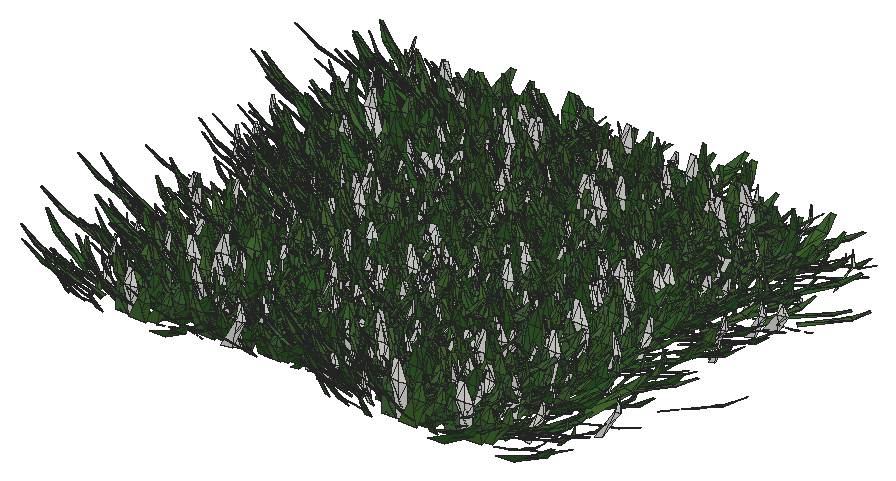
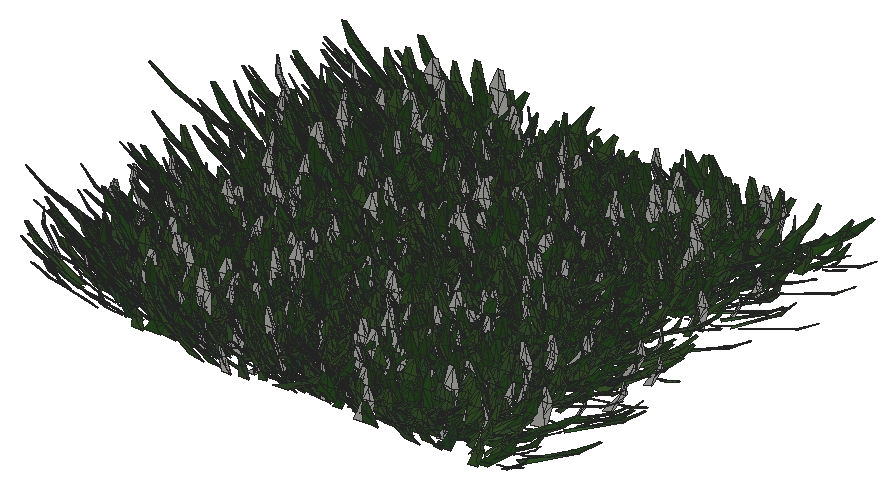
# SketchUp Ruby script. Lengths in inches.
U = 1.inch
M = Sketchup.active_model
def pt(a) = Geom::Point3d.new(a.map { |v| v * U })
def face(e, loops, mat)
  f = e.add_face(loops[0].map { |a| pt(a) })
  loops[1..].each { |l| e.add_face(l.map { |a| pt(a) }).erase! }
  f.material = f.back_material = mat if mat
  f
end
# faces: each face lists its corners as indices into pts; further lists are holes
def faces(e, pts, list, mat = nil) = list.each { |f| face(e, (f[0].is_a?(Array) ? f : [f]).map { |l| l.map { |i| pts[i] } }, mat) }
# xy, xz, yz: faces in a plane at the given z, y or x. An outline is a flat list of corners, or four numbers for a rectangle; further outlines are holes
def ring(l) = l.size == 4 ? [[l[0], l[1]], [l[2], l[1]], [l[2], l[3]], [l[0], l[3]]] : l.each_slice(2).to_a
def flat(e, list, mat, &to3) = list.each { |f| face(e, (f[0].is_a?(Array) ? f : [f]).map { |l| ring(l).map { |u, v| to3.(u, v) } }, mat) }
def xy(e, z, list, mat = nil) = flat(e, list, mat) { |x, y| [x, y, z] }
def xz(e, y, list, mat = nil) = flat(e, list, mat) { |x, z| [x, y, z] }
def yz(e, x, list, mat = nil) = flat(e, list, mat) { |y, z| [x, y, z] }
def lines(e, pts, list) = list.each { |a, b| e.add_line(pt(pts[a]), pt(pts[b])) }
# prism: a flat outline (further loops are holes) pulled along v
def prism(e, loops, v, mat = nil)
  f = face(e, loops, mat); d = Geom::Vector3d.new(v.map { |x| x * U })
  f.pushpull(f.normal.samedirection?(d) ? d.length : -d.length)
end
def box(e, o, s, mat = nil) = prism(e, [[o, [o[0] + s[0], o[1], o[2]], [o[0] + s[0], o[1] + s[1], o[2]], [o[0], o[1] + s[1], o[2]]]], [0, 0, s[2]], mat)
def at(x, y, z, deg = 0) = Geom::Transformation.translation(pt([x, y, z])) * Geom::Transformation.rotation(ORIGIN, Z_AXIS, deg.degrees)
def axes(o, x, y, z) = Geom::Transformation.new([*x, 0, *y, 0, *z, 0, *pt(o).to_a, 1])
def part(name) = M.definitions.add(name)
# library, detail: a bought-in or finely detailed component or shape, given as its bounding box
def library(name, o, s) = part(name).tap { |d| box(d.entities, o, s) }
def detail(e, o, s) = box(e.add_group.entities, o, s)
def put(e, d, t, mat = nil) = e.add_instance(d, t).tap { |i| i.material = mat if mat }
def group(e, t, mat = nil) = e.add_group.tap { |g| g.transformation = t; g.material = mat if mat }.entities
root = M.entities
M.materials.add("Material10").color = [48, 100, 38]
M.materials.add("Material3").color = [68, 110, 58]
M.materials.add("Material4").color = [48, 90, 38]
M.materials.add("Material5").color = [68, 110, 48]
M.materials.add("Material6").color = [48, 90, 48]
M.materials.add("Material7").color = [58, 110, 58]
M.materials.add("Material8").color = [58, 90, 38]
M.materials.add("Material9").color = [68, 100, 58]
c1 = part("grass00")
p = [[-0.6875,0.15,0],[-0.56,0.08,5.52],[-0.04,0.03,2.76],[0.48,-0.02,0],[0.35,-0.02,5.52],[-0.1,-0.14,5.52],
  [-0.12,0.65,8.37],[-0.42,0.65,8.37]]
faces(c1.entities,p,[[0,1,2,3],[3,2,4],[1,5,2],[5,4,2],[1,6,5],[4,5,6],[7,6,1]])
c2 = part("Group16\#1")
put(c2.entities,c1,axes([1.44,-0.61,-0.01],[0.05352,0.12609,0],[-0.10704,0.04543,0.07239],[0.06664,-0.02828,0.11628]),"Material6")
put(c2.entities,c1,axes([0.76,-0.15,-0.01],[0.04676,0.24062,0],[-0.23162,0.04501,0.06642],[0.0652,-0.01267,0.23595]),"Material3")
put(c2.entities,c1,axes([0.79,0.01,-0.01],[-0.00606,0.34651,0],[-0.34381,-0.00602,0.0432],[0.04319,0.00076,0.34386]))
put(c2.entities,c1,axes([1,0.23,-0.01],[-0.07192,0.31144,0],[-0.28722,-0.06632,0.1236],[0.12043,0.02781,0.29478]),"Material5")
put(c2.entities,c1,axes([1.66,0.77,-0.01],[-0.13828,0.29651,0],[-0.21551,-0.1005,0.22471],[0.20365,0.09498,0.23779]),"Material10")
put(c2.entities,c1,axes([0.6875,0.52,-0.01],[-0.18126,0.24051,0],[-0.22746,-0.17142,0.09788],[0.07817,0.05891,0.28481]),"Material5")
put(c2.entities,c1,axes([0.68,0.78,-0.01],[-0.215,0.18688,0],[-0.12385,-0.14248,0.21334],[0.13995,0.16101,0.18878]),"Material3")
put(c2.entities,c1,axes([0.56,1,-0.01],[-0.13756,0.07624,0],[-0.06159,-0.11112,0.0927],[0.04494,0.08108,0.12705]),"Material5")
put(c2.entities,c1,axes([0.2,0.64,-0.01],[-0.23729,0.07254,0],[-0.05711,-0.18681,0.153],[0.04473,0.14632,0.19535]),"Material10")
put(c2.entities,c1,axes([0.0625,0.72,-0.01],[-0.28874,0.02525,0],[-0.02179,-0.24916,0.14647],[0.01276,0.14591,0.25012]),"Material3")
put(c2.entities,c1,axes([-0.08,0.62,-0.01],[-0.34089,-0.04187,0],[0.03255,-0.26504,0.216],[-0.02633,0.21439,0.26703]),"Material10")
put(c2.entities,c1,axes([-0.34,0.98,-0.01],[-0.14314,-0.0493,0],[0.04397,-0.12769,0.06843],[-0.02228,0.0647,0.13505]),"Material10")
put(c2.entities,c1,axes([-0.87,1.45,-0.01],[-0.23488,-0.14114,0],[0.13761,-0.22901,0.06087],[-0.03135,0.05217,0.26717]))
put(c2.entities,c1,axes([-0.72,0.77,-0.01],[-0.14208,-0.13251,0],[0.07209,-0.0773,0.16301],[-0.11118,0.11922,0.1057]),"Material10")
put(c2.entities,c1,axes([-0.62,0.43,-0.01],[-0.14845,-0.21203,0],[0.18654,-0.13061,0.12304],[-0.10079,0.07057,0.22772]),"Material3")
put(c2.entities,c1,axes([-0.68,0.29,-0.01],[-0.13639,-0.32136,0],[0.31723,-0.13464,0.05579],[-0.05136,0.0218,0.34462]),"Material4")
put(c2.entities,c1,axes([-0.64,0.125,-0.01],[-0.0458,-0.23569,0],[0.22124,-0.043,0.08276],[-0.08124,0.01579,0.22538]),"Material7")
put(c2.entities,c1,axes([-1.6,-0.03,-0.01],[0.00576,-0.32897,0],[0.27526,0.00482,0.18018],[-0.18015,-0.00315,0.2753]),"Material5")
put(c2.entities,c1,axes([-1.36,-0.31,-0.01],[0.05718,-0.24765,0],[0.18172,0.04196,0.17267],[-0.16825,-0.03885,0.1865]),"Material10")
put(c2.entities,c1,axes([-1.54,-0.72,-0.01],[0.06537,-0.14017,0],[0.13555,0.06321,0.03939],[-0.0357,-0.01665,0.14956]))
put(c2.entities,c1,axes([-1.19,-0.9,-0.01],[0.09597,-0.12735,0],[0.11214,0.08451,0.07557],[-0.06035,-0.04548,0.14042]),"Material9")
put(c2.entities,c1,axes([-0.47,-0.54,-0.01],[0.11588,-0.10072,0],[0.0618,0.0711,0.12124],[-0.07953,-0.0915,0.0942]))
put(c2.entities,c1,axes([-0.47,-0.84,-0.01],[0.11927,-0.0661,0],[0.06603,0.11913,0.00646],[-0.00313,-0.00565,0.13621]),"Material5")
put(c2.entities,c1,axes([-0.38,-1.24,-0.01],[0.28037,-0.08571,0],[0.0618,0.20215,0.20315],[-0.05939,-0.19428,0.21139]),"Material9")
put(c2.entities,c1,axes([-0.06,-0.66,-0.01],[0.22719,-0.01987,0],[0.01247,0.14255,0.17758],[-0.01547,-0.17691,0.1431]),"Material8")
put(c2.entities,c1,axes([0.11,-0.89,-0.01],[0.14882,0.01828,0],[-0.01058,0.08611,0.12229],[0.01491,-0.12138,0.08676]),"Material6")
put(c2.entities,c1,axes([0.25,-0.72,-0.01],[0.20481,0.07053,0],[-0.06206,0.18022,0.10291],[0.03351,-0.0973,0.1906]),"Material6")
put(c2.entities,c1,axes([0.85,-1.42,-0.01],[0.16481,0.09904,0],[-0.09472,0.15762,0.05616],[0.02893,-0.04814,0.18389]),"Material5")
put(c2.entities,c1,axes([1.01,-1.09,-0.01],[0.21858,0.20385,0],[-0.17495,0.1876,0.15339],[0.10462,-0.11218,0.25652]),"Material10")
put(c2.entities,c1,axes([1.01,-0.71,-0.01],[0.08733,0.12473,0],[-0.06445,0.04512,0.13037],[0.1068,-0.07477,0.07867]),"Material6")
c3 = part("Group15\#1")
put(c3.entities,c2,at(0,0,0))
c4 = part("3darcstudiotree_grass00\#1")
put(c4.entities,c3,at(0,0,0))
put(root,c4,axes([888.68,894.13,0],[0.61281,-1.25792,0],[4.16429,0.12679,-0.0324],[0.1815,0.00553,1.47946]))
put(root,c4,axes([889.35,933.24,0],[-4.67365,-0.16733,0],[0.64986,-1.13441,-0.00988],[0.00864,-0.01508,1.76639]))
put(root,c4,axes([887.89,919.82,0],[-0.28726,1.27917,0],[-3.62125,-0.05083,-0.00552],[-0.03584,-0.0005,1.47331]))
put(root,c4,axes([889.7,899.66,0],[1.5261,-1.19927,0],[4.79938,0.38171,-0.00448],[0.02429,0.00193,1.79011]))
put(root,c4,axes([889.46,902.48,0],[-0.47435,-1.1855,0],[4.17095,-0.10431,-0.05423],[0.34983,-0.00875,1.69842]))
put(root,c4,axes([889.79,918.5,0],[-3.66287,-0.10914,0],[0.53272,-1.11739,-0.01308],[0.00905,-0.01898,1.64432]))
put(root,c4,axes([889.9,927.1,0],[-4.43451,0.03772,0],[-0.16554,-1.21627,-0.01213],[-0.00253,-0.01859,1.86653]))
put(root,c4,axes([889.75,911.6,0],[-3.65887,0.1299,0],[-0.61787,-1.08767,-0.00819],[-0.00564,-0.00993,1.3463]))
put(root,c4,axes([889.55,905.01,0],[-3.669,0.60681,0],[-2.27303,-0.85898,-0.03289],[-0.10969,-0.04145,1.55622]))
put(root,c4,axes([890.45,931.35,0],[-4.28497,-0.45872,0],[1.95501,-1.14138,-0.00601],[0.01191,-0.00695,1.5624]))
put(root,c4,axes([890.35,908.66,0],[-3.05739,-0.71664,0],[2.47729,-0.66055,-0.04465],[0.23187,-0.06183,1.71883]))
put(root,c4,axes([890.83,895.05,0],[-4.36075,-0.60413,0],[2.40015,-1.0828,-0.02403],[0.07228,-0.03261,1.92026]))
put(root,c4,axes([888.54,915.54,0],[3.04221,0.50388,0],[-2.77722,1.04797,-0.00365],[-0.00864,0.00326,1.34685]))
put(root,c4,axes([889.4375,925.43,0],[4.61314,0.2073,0],[-0.8279,1.1515,-0.00017],[-0.00019,0.00026,1.78268]))
put(root,c4,axes([891.2,898.44,0],[-2.44705,-0.6793,0],[3.03744,-0.68387,-0.04825],[0.26014,-0.05857,1.85346]))
put(root,c4,axes([890.42,923.9,0],[-2.92283,0.91805,0],[-3.29129,-0.65491,-0.02078],[-0.1142,-0.02272,1.84714]))
put(root,c4,axes([889.58,905.98,0],[4.43029,0.19931,0],[-0.91399,1.26978,-0.01866],[-0.01759,0.02444,1.717]))
put(root,c4,axes([889.93,921.08,0],[3.52512,0.8325,0],[-3.53899,0.93659,-0.01632],[-0.05093,0.01348,1.46423]))
put(root,c4,axes([890.42,916.13,0],[3.74573,0.67429,0],[-2.32637,0.8077,-0.02682],[-0.11092,0.03851,1.76121]))
put(root,c4,axes([891.78,930.35,0],[-1.7815,0.94038,0],[-4.05374,-0.47998,-0.05633],[-0.34181,-0.04047,1.88219]))
put(root,c4,axes([891.42,913.95,0],[2.43331,0.85712,0],[-3.60269,0.63924,-0.0048],[-0.0225,0.00399,1.58899]))
put(root,c4,axes([893.59,904.56,0],[-3.5004,-0.31733,0],[1.33107,-0.91766,-0.00444],[0.00863,-0.00595,1.39182]))
put(root,c4,axes([894.39,922.36,0],[0.98634,-0.98273,0],[4.96113,0.31121,-0.03647],[0.15012,0.00942,1.35653]))
put(root,c4,axes([894.27,931.77,0],[1.5516,-0.99587,0],[4.11909,0.4011,-0.0174],[0.07644,0.00744,1.30214]))
put(root,c4,axes([894.18,913.87,0],[1.28741,-1.026,0],[3.77436,0.296,-0.02865],[0.19326,0.01516,1.74795]))
put(root,c4,axes([893.8,903.46,0],[2.57556,-0.96136,0],[3.42516,0.57352,-0.05113],[0.25858,0.0433,1.56833]))
put(root,c4,axes([894.82,900.16,0],[0.62856,-1.17531,0],[4.83812,0.16171,-0.0102],[0.05862,0.00196,1.76846]))
put(root,c4,axes([895.13,907.88,0],[-3.61051,-0.41144,0],[1.52061,-0.83398,-0.0331],[0.09259,-0.05078,1.54531]))
put(root,c4,axes([893.88,905.65,0],[2.93142,0.86988,0],[-2.89804,0.61038,-0.04423],[-0.19713,0.04152,1.38013]))
put(root,c4,axes([895.13,921.54,0],[2.02846,-0.79273,0],[3.7574,0.60091,-0.02581],[0.12575,0.02011,1.61243]))
put(root,c4,axes([895.68,915.18,0],[-0.79202,-1.12645,0],[4.16541,-0.18305,-0.04893],[0.31505,-0.01384,1.72817]))
put(root,c4,axes([895.39,930.26,0],[-4.0818,0.563,0],[-2.02545,-0.91779,-0.01481],[-0.0392,-0.01776,1.43556]))
put(root,c4,axes([894.68,924.47,0],[4.56829,-0.12289,0],[0.55043,1.27888,-0.03237],[0.01647,0.03827,1.52951]))
put(root,c4,axes([896.36,901.64,0],[-4.66423,-0.46806,0],[1.3813,-0.8603,-0.04034],[0.1029,-0.06409,1.58691]))
put(root,c4,axes([896.29,919.56,0],[-0.8253,-1.0659,0],[3.55539,-0.17205,-0.00678],[0.0454,-0.0022,1.54322]))
put(root,c4,axes([896.8,917.01,0],[-2.41791,-1.09567,0],[4.13972,-0.57097,-0.0117],[0.05943,-0.0082,1.7149]))
put(root,c4,axes([895.04,932.84,0],[1.31705,0.88702,0],[-3.52607,0.32722,-0.04291],[-0.24696,0.02292,1.44315]))
put(root,c4,axes([895.89,927.84,0],[2.84794,-0.83805,0],[3.51838,0.74728,-0.02612],[0.12969,0.02754,1.8801]))
put(root,c4,axes([895.27,895.97,0],[-0.36246,1.18288,0],[-4.29439,-0.08224,-0.03234],[-0.22764,-0.00436,1.90052]))
put(root,c4,axes([894.93,917.92,0],[4.24178,0.73433,0],[-2.3441,0.84628,-0.05103],[-0.19051,0.06878,1.6877]))
put(root,c4,axes([895.36,896.54,0],[4.6373,-0.30696,0],[1.13066,1.06758,-0.03329],[0.04185,0.03952,1.35616]))
put(root,c4,axes([896.33,898.9375,0],[-3.30831,0.84443,0],[-3.70005,-0.906,-0.0181],[-0.07733,-0.01894,1.93624]))
put(root,c4,axes([897.11,909.39,0],[1.24763,-0.92182,0],[4.38061,0.37056,-0.02846],[0.12558,0.01062,1.34635]))
put(root,c4,axes([897.625,910.63,0],[1.57584,-0.93457,0],[3.47629,0.36635,-0.03331],[0.19752,0.02082,1.51731]))
put(root,c4,axes([897.64,925.62,0],[-2.4775,0.7659,0],[-2.94091,-0.59457,-0.00747],[-0.03328,-0.00673,1.35493]))
put(root,c4,axes([897.78,929.1875,0],[0.67051,0.95222,0],[-4.84197,0.21309,-0.06022],[-0.34411,0.01514,1.78296]))
put(root,c4,axes([897.8,911.56,0],[2.1541,0.73783,0],[-3.48209,0.63537,-0.05552],[-0.23217,0.04236,1.39481]))
put(root,c4,axes([899.92,932.08,0],[-1.49369,-1.06151,0],[3.72951,-0.32799,-0.03242],[0.16562,-0.01457,1.33794]))
put(root,c4,axes([901.23,895.25,0],[-4.2486,-0.47023,0],[1.56425,-0.88333,-0.0129],[0.02854,-0.01611,1.31952]))
put(root,c4,axes([900.17,922.18,0],[-3.0514,0.75193,0],[-3.33727,-0.84644,-0.00446],[-0.01526,-0.00387,1.44777]))
put(root,c4,axes([901.21,913.16,0],[-4.92331,0.15002,0],[-0.48598,-0.99677,-0.03065],[-0.02921,-0.05991,1.97713]))
put(root,c4,axes([901.76,929.9375,0],[-1.91157,-1.00019,0],[4.33506,-0.51782,-0.00689],[0.03608,-0.00431,1.74288]))
put(root,c4,axes([901.7,926.82,0],[-3.45228,-0.31834,0],[1.71903,-1.16515,-0.02933],[0.05627,-0.03814,1.72129]))
put(root,c4,axes([900.31,932.9,0],[4.75785,0.13927,0],[-0.57992,1.23828,-0.02723],[-0.01633,0.03486,1.60719]))
put(root,c4,axes([900.73,898.41,0],[4.24363,-0.133,0],[0.6088,1.21409,-0.03701],[0.03003,0.05988,1.99511]))
put(root,c4,axes([900.46,917.24,0],[4.38323,0.5518,0],[-2.13593,1.06042,-0.03278],[-0.09357,0.04645,1.8841]))
put(root,c4,axes([901.91,912.36,0],[1.80526,-0.93773,0],[4.63497,0.55769,-0.06017],[0.29336,0.0353,1.73941]))
put(root,c4,axes([901.75,905.75,0],[2.55214,-0.79924,0],[2.90871,0.58051,-0.01018],[0.05177,0.01033,1.51436]))
put(root,c4,axes([900.92,924.17,0],[3.99552,0.1688,0],[-0.66851,0.98901,-0.04218],[-0.052,0.07693,1.85529]))
put(root,c4,axes([902.54,902.82,0],[-1.20745,-0.91696,0],[4.5972,-0.37835,-0.05688],[0.32578,-0.02681,1.82396]))
put(root,c4,axes([900.85,909.42,0],[4.60083,0.27128,0],[-0.99888,1.0588,-0.02883],[-0.04481,0.04749,1.84132]))
put(root,c4,axes([901.9375,901.72,0],[3.15828,-0.63994,0],[3.01444,0.92981,-0.02341],[0.07838,0.02418,1.59067]))
put(root,c4,axes([903.11,918.12,0],[-3.6011,-0.51295,0],[1.91228,-0.83905,-0.01205],[0.03293,-0.01445,1.33255]))
put(root,c4,axes([903.23,904.54,0],[-3.34758,-0.57583,0],[2.35115,-0.85428,-0.02104],[0.0798,-0.02899,1.73448]))
put(root,c4,axes([903.24,925.52,0],[-2.89247,-0.63047,0],[2.79907,-0.8026,-0.03875],[0.16322,-0.0468,1.70607]))
put(root,c4,axes([902.44,907.57,0],[2.73531,-0.60508,0],[3.15346,0.89096,-0.04815],[0.2108,0.05956,1.9649]))
put(root,c4,axes([902.18,928.46,0],[3.9102,0.44615,0],[-1.54008,0.84362,-0.03533],[-0.11802,0.06465,1.86502]))
put(root,c4,axes([903.1,915.37,0],[4.11404,0.2026,0],[-0.94809,1.20329,-0.03192],[-0.02927,0.03715,1.45488]))
put(root,c4,axes([903.49,920.89,0],[-0.49166,1.00113,0],[-4.41418,-0.13549,-0.03564],[-0.21762,-0.00668,1.71014]))
put(root,c4,axes([903.1,899.47,0],[4.50169,0.36178,0],[-1.23301,0.95889,-0.00634],[-0.01342,0.01044,1.74238]))
put(root,c4,axes([904.07,910.4,0],[3.54844,-0.68412,0],[2.53941,0.82322,-0.00737],[0.02478,0.00803,1.42978]))
put(root,c4,axes([903.35,896.59,0],[0.51658,1.03873,0],[-3.86244,0.12005,-0.00588],[-0.03275,0.00102,1.36568]))
put(root,c4,axes([903.26,920,0],[2.79958,0.75017,0],[-3.79275,0.88464,-0.03325],[-0.11995,0.02798,1.59934]))
put(root,c4,axes([905.78,931.97,0],[-3.89596,-0.25813,0],[1.01122,-0.9539,-0.01321],[0.02668,-0.02516,1.9444]))
put(root,c4,axes([906.1,909.61,0],[-1.738,-0.84913,0],[4.25665,-0.54453,-0.02541],[0.1,-0.01279,1.32108]))
put(root,c4,axes([905.89,921.55,0],[0.41155,-0.92389,0],[4.43873,0.12358,-0.00391],[0.01942,0.00054,1.39627]))
put(root,c4,axes([905.66,917.17,0],[0.3191,-1.2505,0],[4.37865,0.06983,-0.05413],[0.27394,0.00437,1.39055]))
put(root,c4,axes([905.87,907.09,0],[0.66073,-1.27721,0],[5.08368,0.16437,-0.05291],[0.21846,0.00706,1.33374]))
put(root,c4,axes([906.14,901.94,0],[-4.56571,-0.14579,0],[0.54682,-1.07027,-0.0157],[0.01423,-0.02784,1.92971]))
put(root,c4,axes([906.22,930.68,0],[0.35405,-1.11937,0],[4.05484,0.08016,-0.00365],[0.02209,0.00044,1.54435]))
put(root,c4,axes([906.28,915.22,0],[2.95951,-0.93197,0],[4.0202,0.79789,-0.06314],[0.20058,0.03981,1.30132]))
put(root,c4,axes([906.46,900.2,0],[-3.85049,0.40649,0],[-1.93296,-1.14436,-0.01449],[-0.02989,-0.0177,1.64714]))
put(root,c4,axes([907.85,933.38,0],[-2.15911,-0.91358,0],[4.38085,-0.64709,-0.05519],[0.27113,-0.04005,1.81465]))
put(root,c4,axes([905.8125,910.7,0],[2.25416,0.91391,0],[-3.32067,0.5119,-0.00763],[-0.0422,0.0065,1.58363]))
put(root,c4,axes([906.26,919.56,0],[4.35171,-0.00299,0],[0.0127,1.15651,-0.02008],[0.00031,0.02806,1.61638]))
put(root,c4,axes([906.39,903.58,0],[0.76881,0.99481,0],[-3.92404,0.18954,-0.03785],[-0.21203,0.01024,1.42505]))
put(root,c4,axes([908.21,928.39,0],[-3.65156,-0.16407,0],[0.77449,-1.07733,-0.01818],[0.01589,-0.02211,1.35222]))
put(root,c4,axes([908.57,906.01,0],[-4.40837,-0.63137,0],[2.29025,-0.99943,-0.04075],[0.1094,-0.04774,1.55523]))
put(root,c4,axes([906.54,918.55,0],[4.60532,0.48375,0],[-1.62275,0.96554,-0.00848],[-0.02401,0.01429,1.91304]))
put(root,c4,axes([906.77,904.74,0],[4.22855,0.37749,0],[-1.56983,1.09905,-0.00059],[-0.00119,0.00083,1.74794]))
put(root,c4,axes([908.26,924.16,0],[2.56038,-0.8827,0],[3.78234,0.6857,-0.00976],[0.05125,0.00929,1.89325]))
put(root,c4,axes([908.62,925.48,0],[-0.92872,-0.91526,0],[4.23097,-0.26832,-0.05601],[0.35873,-0.02275,1.80254]))
put(root,c4,axes([908.63,914.12,0],[2.77364,-0.77685,0],[3.77594,0.8426,-0.02458],[0.10362,0.02312,1.78746]))
put(root,c4,axes([909.72,922.93,0],[-4.1547,-0.33584,0],[1.51583,-1.17203,-0.04655],[0.07348,-0.05682,1.58019]))
put(root,c4,axes([908.33,898.25,0],[3.93015,-0.3044,0],[1.10624,0.89267,-0.04073],[0.07417,0.05985,1.43775]))
put(root,c4,axes([908.37,897.09,0],[1.67946,0.90749,0],[-4.52669,0.52358,-0.03574],[-0.19906,0.02302,1.91331]))
put(root,c4,axes([908.86,927.43,0],[4.66183,0.56246,0],[-1.8815,0.97465,-0.05424],[-0.11893,0.06161,1.36476]))
put(root,c4,axes([910.12,911.71,0],[1.39071,-1.04081,0],[3.42496,0.28602,-0.03453],[0.25559,0.02134,1.76116]))
put(root,c4,axes([910.18,895.9,0],[0.96858,0.89112,0],[-3.74023,0.25408,-0.02204],[-0.16423,0.01116,1.87051]))
put(root,c4,axes([911.91,905.84,0],[-4.69188,-0.0249,0],[0.0963,-1.13384,-0.04949],[0.00708,-0.08333,1.9102]))
put(root,c4,axes([912.98,926.27,0],[-1.9675,-0.8496,0],[3.8564,-0.55817,-0.02105],[0.1271,-0.0184,1.94345]))
put(root,c4,axes([912.09,924.29,0],[-3.4865,0.64506,0],[-2.72844,-0.92168,-0.01624],[-0.06139,-0.02074,1.82169]))
put(root,c4,axes([912.58,910.07,0],[2.44226,-0.75549,0],[3.06681,0.61963,-0.01488],[0.06384,0.0129,1.35946]))
put(root,c4,axes([913.45,922.65,0],[-2.44027,-0.95657,0],[3.80591,-0.60682,-0.04256],[0.19819,-0.0316,1.55835]))
put(root,c4,axes([912.11,930.61,0],[3.65585,-0.02969,0],[0.16476,1.26817,-0.05593],[0.00918,0.07069,1.60461]))
put(root,c4,axes([913.58,928.44,0],[0.86009,-1.01814,0],[4.02529,0.21253,-0.00249],[0.01488,0.00079,1.57305]))
put(root,c4,axes([914.11,932.19,0],[-0.68955,-0.89341,0],[4.9756,-0.24002,-0.02161],[0.13108,-0.00632,1.95654]))
put(root,c4,axes([913.84,902.87,0],[1.44071,-0.87984,0],[4.07175,0.41671,-0.00546],[0.02449,0.00251,1.33158]))
put(root,c4,axes([912.47,919.94,0],[1.00747,0.90236,0],[-3.56805,0.24898,-0.02635],[-0.15857,0.01106,1.4463]))
put(root,c4,axes([912.94,927.17,0],[-2.23722,1.02937,0],[-4.10468,-0.55756,-0.0267],[-0.10588,-0.01438,1.31753]))
put(root,c4,axes([914.2,894.18,0],[1.23489,-1.20152,0],[4.58168,0.29431,-0.01129],[0.06903,0.00443,1.86628]))
put(root,c4,axes([912.5,918.32,0],[4.08208,0.66427,0],[-2.13929,0.82165,-0.02904],[-0.11461,0.04402,1.7729]))
put(root,c4,axes([913.3,916.31,0],[3.71734,-0.40813,0],[1.8446,1.05006,-0.00525],[0.01214,0.00691,1.64886]))
put(root,c4,axes([913.47,920.82,0],[3.61412,-0.47878,0],[2.26101,1.06672,-0.00115],[0.00254,0.0012,1.42878]))
put(root,c4,axes([912.91,907.99,0],[3.34943,0.40768,0],[-2.23658,1.14845,-0.05845],[-0.12336,0.06334,1.53958]))
put(root,c4,axes([914.74,901.31,0],[-4.90262,0.38062,0],[-1.21174,-0.97549,-0.03919],[-0.07726,-0.06219,1.69748]))
put(root,c4,axes([913.5,913.76,0],[4.40316,-0.08214,0],[0.30096,1.00833,-0.02534],[0.0118,0.03954,1.58232]))
put(root,c4,axes([914.11,897.42,0],[3.91548,-0.26914,0],[1.03869,0.94445,-0.03828],[0.06514,0.05923,1.57185]))
put(root,c4,axes([913.93,915.7,0],[4.05806,0.27476,0],[-1.0531,0.97211,-0.0432],[-0.06805,0.06282,1.51727]))
put(root,c4,axes([914.75,898.76,0],[-2.36017,0.90935,0],[-3.92025,-0.63593,-0.05659],[-0.22736,-0.03688,1.39892]))
put(root,c4,axes([915.93,912.21,0],[3.07578,-0.55136,0],[2.5802,0.89961,-0.04704],[0.16898,0.05892,1.70604]))
put(root,c4,axes([915.04,895.46,0],[3.3125,0.68522,0],[-3.11487,0.94112,-0.00662],[-0.02265,0.00684,1.63949]))
put(root,c4,axes([915.93,908.83,0],[4.72223,0.15279,0],[-0.65977,1.27445,-0.04718],[-0.02776,0.05361,1.4726]))
put(root,c4,axes([916.22,900.04,0],[0.9264,1.21479,0],[-3.78487,0.1804,-0.03349],[-0.21957,0.01047,1.60736]))
put(root,c4,axes([917.86,900.57,0],[-3.0009,-0.56917,0],[2.28303,-0.75232,-0.01586],[0.06179,-0.02036,1.52204]))
put(root,c4,axes([916.1875,904.6875,0],[4.12875,0.54518,0],[-1.92192,0.90969,-0.05015],[-0.16609,0.07861,1.82381]))
put(root,c4,axes([917.87,914.1875,0],[3.49538,-0.78655,0],[2.6672,0.74081,-0.02235],[0.11606,0.03224,1.93391]))
put(root,c4,axes([918.56,918.69,0],[2.53666,-1.01382,0],[4.04089,0.63191,-0.01393],[0.05733,0.00897,1.44657]))
put(root,c4,axes([918.62,932.17,0],[-4.33002,0.49068,0],[-1.86161,-1.02674,-0.00714],[-0.01364,-0.00752,1.30481]))
put(root,c4,axes([918.92,909.33,0],[2.06526,-1.11645,0],[4.68232,0.54135,-0.01],[0.05596,0.00647,1.98774]))
put(root,c4,axes([918.0625,907.96,0],[-2.02693,0.82712,0],[-3.18296,-0.48751,-0.01687],[-0.08389,-0.01285,1.36079]))
put(root,c4,axes([919.42,895.1,0],[1.53918,-1.14465,0],[4.66766,0.39228,-0.02131],[0.11149,0.00937,1.69918]))
put(root,c4,axes([918.72,904.86,0],[2.64191,-0.97906,0],[3.33396,0.56227,-0.04469],[0.26935,0.04543,1.8275]))
put(root,c4,axes([919.93,916.91,0],[-3.19126,-0.77471,0],[2.91337,-0.75007,-0.03796],[0.16003,-0.0412,1.58175]))
put(root,c4,axes([918.22,927.06,0],[-0.05785,0.90621,0],[-4.99492,-0.01993,-0.04794],[-0.2528,-0.00101,1.64652]))
put(root,c4,axes([919.41,919.14,0],[1.75969,-1.05403,0],[3.90588,0.40755,-0.05171],[0.2964,0.03093,1.64301]))
put(root,c4,axes([920.66,929.11,0],[-1.78532,-1.2019,0],[4.51139,-0.41883,-0.00006],[0.00036,-0.00003,1.81412]))
put(root,c4,axes([918.87,929.99,0],[0.51329,0.95207,0],[-4.68245,0.15778,-0.05207],[-0.31247,0.01053,1.7882]))
put(root,c4,axes([920.63,901.16,0],[-3.2892,-0.91562,0],[3.69199,-0.82892,-0.05274],[0.25135,-0.05643,1.98669]))
put(root,c4,axes([918.83,897.25,0],[1.0775,1.11347,0],[-4.72291,0.28565,-0.01063],[-0.05061,0.00306,1.48723]))
put(root,c4,axes([919.68,925.4,0],[4.44444,0.2645,0],[-1.11366,1.16958,-0.06215],[-0.07819,0.08211,1.63292]))
put(root,c4,axes([921.67,921.02,0],[-3.61007,-0.50137,0],[2.38008,-1.07109,-0.02959],[0.07743,-0.03484,1.65043]))
put(root,c4,axes([919.93,924.38,0],[1.61493,0.96375,0],[-4.19905,0.43976,-0.03717],[-0.19495,0.02042,1.61797]))
put(root,c4,axes([919.94,910.64,0],[3.19389,0.68135,0],[-2.76112,0.80894,-0.03219],[-0.14851,0.04351,1.88986]))
put(root,c4,axes([919.71,898.03,0],[2.54006,0.86329,0],[-3.88327,0.71411,-0.02079],[-0.07531,0.01385,1.35493]))
put(root,c4,axes([922.13,922.89,0],[-4.83306,-0.46342,0],[1.78522,-1.16366,-0.02874],[0.04422,-0.02883,1.33872]))
put(root,c4,axes([921.55,915.46,0],[-2.9698,0.72084,0],[-3.26499,-0.84071,-0.01854],[-0.07852,-0.02022,1.78092]))
put(root,c4,axes([921.53,906.38,0],[4.49031,-0.36697,0],[1.37458,1.05122,-0.04269],[0.09285,0.07101,1.93529]))
